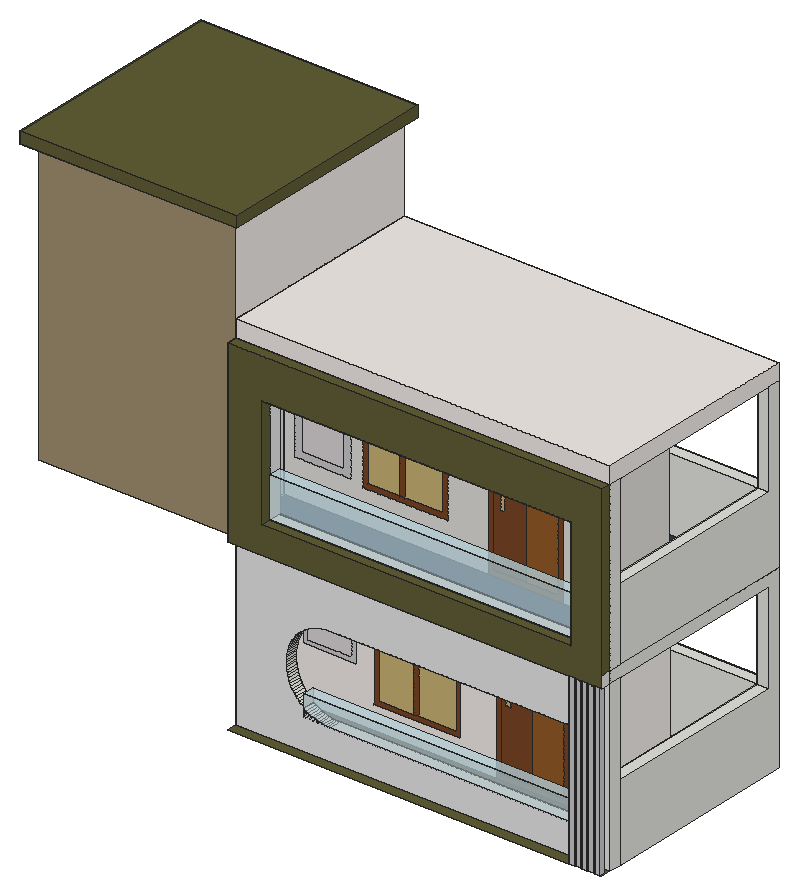
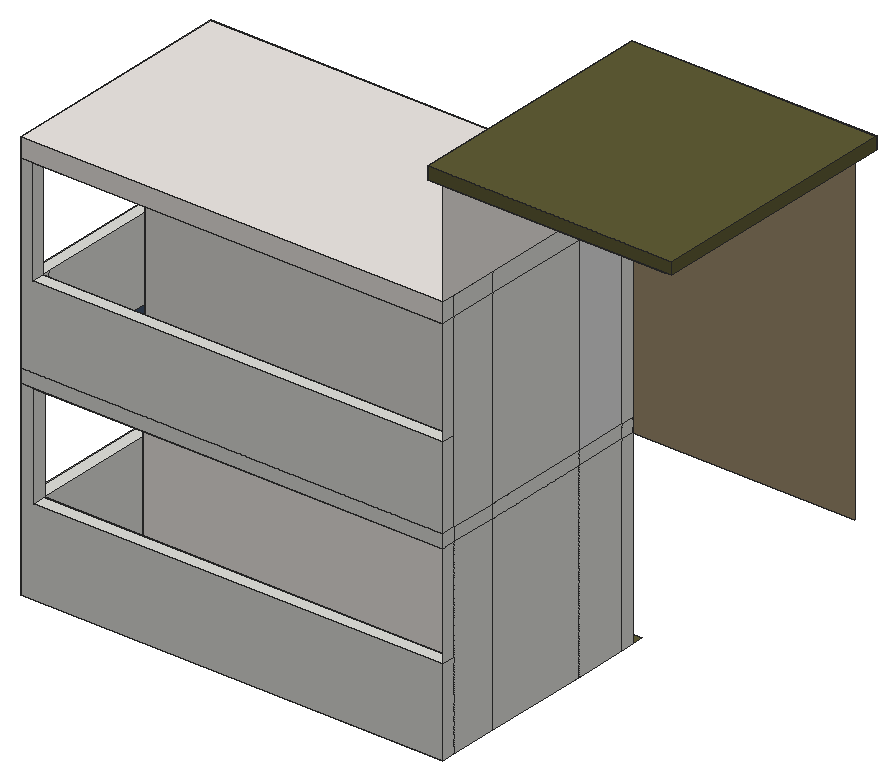
# SketchUp Ruby script. Lengths in inches.
U = 1.inch
M = Sketchup.active_model
def pt(a) = Geom::Point3d.new(a.map { |v| v * U })
def face(e, loops, mat)
  f = e.add_face(loops[0].map { |a| pt(a) })
  loops[1..].each { |l| e.add_face(l.map { |a| pt(a) }).erase! }
  f.material = f.back_material = mat if mat
  f
end
# faces: each face lists its corners as indices into pts; further lists are holes
def faces(e, pts, list, mat = nil) = list.each { |f| face(e, (f[0].is_a?(Array) ? f : [f]).map { |l| l.map { |i| pts[i] } }, mat) }
# xy, xz, yz: faces in a plane at the given z, y or x. An outline is a flat list of corners, or four numbers for a rectangle; further outlines are holes
def ring(l) = l.size == 4 ? [[l[0], l[1]], [l[2], l[1]], [l[2], l[3]], [l[0], l[3]]] : l.each_slice(2).to_a
def flat(e, list, mat, &to3) = list.each { |f| face(e, (f[0].is_a?(Array) ? f : [f]).map { |l| ring(l).map { |u, v| to3.(u, v) } }, mat) }
def xy(e, z, list, mat = nil) = flat(e, list, mat) { |x, y| [x, y, z] }
def xz(e, y, list, mat = nil) = flat(e, list, mat) { |x, z| [x, y, z] }
def yz(e, x, list, mat = nil) = flat(e, list, mat) { |y, z| [x, y, z] }
def lines(e, pts, list) = list.each { |a, b| e.add_line(pt(pts[a]), pt(pts[b])) }
# prism: a flat outline (further loops are holes) pulled along v
def prism(e, loops, v, mat = nil)
  f = face(e, loops, mat); d = Geom::Vector3d.new(v.map { |x| x * U })
  f.pushpull(f.normal.samedirection?(d) ? d.length : -d.length)
end
def box(e, o, s, mat = nil) = prism(e, [[o, [o[0] + s[0], o[1], o[2]], [o[0] + s[0], o[1] + s[1], o[2]], [o[0], o[1] + s[1], o[2]]]], [0, 0, s[2]], mat)
def at(x, y, z, deg = 0) = Geom::Transformation.translation(pt([x, y, z])) * Geom::Transformation.rotation(ORIGIN, Z_AXIS, deg.degrees)
def axes(o, x, y, z) = Geom::Transformation.new([*x, 0, *y, 0, *z, 0, *pt(o).to_a, 1])
def part(name) = M.definitions.add(name)
# library, detail: a bought-in or finely detailed component or shape, given as its bounding box
def library(name, o, s) = part(name).tap { |d| box(d.entities, o, s) }
def detail(e, o, s) = box(e.add_group.entities, o, s)
def put(e, d, t, mat = nil) = e.add_instance(d, t).tap { |i| i.material = mat if mat }
def group(e, t, mat = nil) = e.add_group.tap { |g| g.transformation = t; g.material = mat if mat }.entities
root = M.entities
M.materials.add("[0057_DarkKhaki]").color = [96, 93, 54]
M.materials.add("[Blinds Cellular White]").color = [217, 211, 213]
M.materials.add("[Leather Blue]").color = [45, 57, 74]
M.materials.add("[Leather Red Brown]").color = [76, 40, 8]
M.materials.add("[Polished Concrete New]").color = [200, 200, 203]
M.materials.add("[Polished Concrete Old]").color = [229, 229, 229]
M.materials.add("[Terrazzo Tile Accent]").color = [224, 221, 217]
M.materials.add("[Tile Border Travertine]").color = [160, 142, 112]
M.materials.add("[Translucent Glass Safety]").color = [204, 235, 244]
M.materials["[Translucent Glass Safety]"].alpha = 0.5
M.materials.add("[White Square Tile]").color = [240, 234, 230]
M.materials.add("[Window Covering 02]").color = [199, 178, 115]
M.materials.add("[Wood Floor Light]").color = [204, 176, 127]
M.materials.add("[Wood Floor Parquet]").color = [145, 89, 39]
M.materials.add("[Wood Veneer 01]").color = [120, 70, 37]
xy(root,986.8125,[[1036.87,294.37,1047.2,304.24],[1049.06,294.37,1059.38,304.24],[1060.68,294.37,1071.01,304.24],[1073.18,294.37,1083.51,304.24],[1085.87,294.37,1096.2,304.24],
  [386.67,314.12,1099.23,336.81],[1076.54,336.81,1076.54,692.27,386.67,692.27,386.67,714.96,1099.23,714.96,1099.23,336.81],[386.67,429.17,977.4,609.95]])
xy(root,986.8125,[[386.67,294.37,1036.87,294.37,1036.87,304.24,1047.2,304.24,1047.2,294.37,1049.06,294.37,1049.06,304.24,1059.38,304.24,1059.38,294.37,1060.68,294.37,1060.68,304.24,1071.01,304.24,1071.01,294.37,1073.18,294.37,1073.18,304.24,1083.51,304.24,1083.51,294.37,1085.87,294.37,1085.87,304.24,1096.2,304.24,1096.2,294.37,1099.23,294.37,1099.23,314.12,386.67,314.12]],"[0057_DarkKhaki]")
xy(root,986.8125,[[386.67,336.81,1076.54,336.81,1076.54,692.27,386.67,692.27,386.67,609.95,977.4,609.95,977.4,429.17,386.67,429.17]],"[Leather Red Brown]")
xy(root,1044.74,[[515.75,314.12,565.62,336.81],[565.62,314.12,1076.54,336.81]])
xy(root,1084.42,[[515.75,314.12,1076.54,336.81]],"[Translucent Glass Safety]")
xy(root,1132.25,[[1076.54,336.81,1099.23,692.27],[386.67,692.27,1076.54,714.96]])
xy(root,1210.05,[[565.62,314.12,1076.54,336.81]])
xy(root,1306.5625,[[1036.87,294.37,1047.2,295.05],[1049.06,294.37,1059.38,295.05],[1060.68,294.37,1071.01,295.05],[1073.18,294.37,1083.51,295.05],[1085.87,294.37,1096.2,295.05],
  [386.67,295.05,977.4,314.12],[977.4,295.05,977.4,314.12,1076.54,314.12,1076.54,304.24,1073.18,304.24,1073.18,295.05,1071.01,295.05,1071.01,304.24,1060.68,304.24,1060.68,295.05,1059.38,295.05,1059.38,304.24,1049.06,304.24,1049.06,295.05,1047.2,295.05,1047.2,304.24,1036.87,304.24,1036.87,295.05],[1036.87,295.05,1047.2,304.24],[1049.06,295.05,1059.38,304.24],[1060.68,295.05,1071.01,304.24],
  [1073.18,295.05,1076.54,304.24],[1076.54,295.05,1083.51,304.24],[1083.51,295.05,1083.51,304.24,1076.54,304.24,1076.54,314.12,1099.23,314.12,1099.23,295.05,1096.2,295.05,1096.2,304.24,1085.87,304.24,1085.87,295.05],[1085.87,295.05,1096.2,304.24],[386.67,314.12,977.4,336.81],
  [977.4,314.12,1076.54,336.81],[1076.54,314.12,1099.23,336.81],[386.67,336.81,1099.23,429.17],[386.67,429.17,977.4,609.95],[977.4,429.17,977.4,714.96,1076.54,714.96,1076.54,692.27,1099.23,692.27,1099.23,429.17],
  [386.67,609.95,977.4,714.96]])
xy(root,1329.25,[[1078.73,336.81,1078.73,692.27,386.67,692.27,386.67,714.96,1099.23,714.96,1099.23,336.81],[386.67,429.17,973.89,609.95]])
xy(root,1329.25,[[386.67,336.81,1078.73,336.81,1078.73,692.27,386.67,692.27,386.67,609.95,973.89,609.95,973.89,429.17,386.67,429.17]],"[Leather Blue]")
xy(root,1358.875,[[451.45,314.12,1039.41,336.81]])
xy(root,1358.875,[[451.45,295.05,1039.41,314.12]],"[0057_DarkKhaki]")
xy(root,1436.0625,[[451.45,314.12,1039.41,336.81]],"[Translucent Glass Safety]")
xy(root,1467.875,[[1078.73,336.81,1099.23,692.27],[386.67,692.27,1078.73,714.96]])
xy(root,1571.07,[[451.45,314.12,1039.41,336.81]])
xy(root,1571.07,[[451.45,295.05,1039.41,314.12]],"[0057_DarkKhaki]")
xy(root,1646.9375,[[386.67,336.81,1099.23,429.17],[386.67,429.17,973.89,609.95],[973.89,429.17,973.89,714.96,1078.73,714.96,1078.73,692.27,1099.23,692.27,1099.23,429.17],[386.67,609.95,973.89,714.96],[1078.73,692.27,1099.23,714.96]])
xy(root,1646.9375,[[386.67,295.05,1099.23,314.12]],"[0057_DarkKhaki]")
xy(root,1679.125,[[386.67,314.12,1099.23,714.96]],"[White Square Tile]")
xy(root,1855.8125,[[11.875,314.12,386.67,714.96]])
xy(root,1855.8125,[[0,284.3,0,314.12,386.67,314.12,386.67,714.96,412.48,714.96,412.48,284.3],[0,314.12,11.875,714.96]],"[0057_DarkKhaki]")
xy(root,1876.625,[[0,284.3,412.48,714.96]],"[0057_DarkKhaki]")
xz(root,284.3,[[0,1855.8125,412.48,1876.625]],"[0057_DarkKhaki]")
xz(root,294.37,[[1036.87,986.8125,1047.2,1306.5625],[1049.06,986.8125,1059.38,1306.5625],[1060.68,986.8125,1071.01,1306.5625],[1073.18,986.8125,1083.51,1306.5625],[1085.87,986.8125,1096.2,1306.5625]],"[Polished Concrete New]")
xz(root,295.05,[[[386.67,1306.5625,1099.23,1646.9375],[451.45,1358.875,1039.41,1571.07]]],"[0057_DarkKhaki]")
xz(root,304.24,[[1036.87,986.8125,1047.2,1306.5625],[1049.06,986.8125,1059.38,1306.5625],[1060.68,986.8125,1071.01,1306.5625],[1073.18,986.8125,1083.51,1306.5625],[1085.87,986.8125,1096.2,1306.5625]])
xz(root,314.12,[[515.75,1044.74,565.62,1044.74,561.3,1044.85,556.98,1045.1875,552.69,1045.75,548.4375,1046.54,544.23,1047.55,540.08,1048.78,538.62,1049.3,515.75,1049.3],[515.75,1049.3,538.62,1049.3,536,1050.23,532,1051.88,528.1,1053.74,524.29,1055.81,520.6,1058.07,517.04,1060.52,515.75,1061.51],[[386.67,1306.5625,1099.23,1646.9375],[451.45,1358.875,1039.41,1571.07]]])
xz(root,314.12,[[[386.67,986.8125,1099.23,1306.5625],[565.62,1044.74,561.3,1044.85,556.98,1045.1875,552.69,1045.75,548.4375,1046.54,544.23,1047.55,540.08,1048.78,538.62,1049.3,536,1050.23,532,1051.88,528.1,1053.74,524.29,1055.81,520.6,1058.07,517.04,1060.52,513.6,1063.16,510.3125,1065.97,507.17,1068.94,504.2,1072.08,501.38,1075.375,498.75,1078.81,496.3,1082.375,494.04,1086.0625,491.97,1089.87,490.11,1093.77,488.45,1097.77,487.01,1101.85,485.78,1106,484.77,1110.21,483.98,1114.46,483.42,1118.75,483.08,1123.07,482.96,1127.39,483.08,1131.72,483.42,1136.03,483.98,1140.32,484.77,1144.58,485.78,1148.78,487.01,1152.93,488.45,1157.01,490.11,1161.01,491.97,1164.92,494.04,1168.72,496.3,1172.41,498.75,1175.98,501.38,1179.41,504.2,1182.7,507.17,1185.84,510.3125,1188.82,513.6,1191.63,517.04,1194.26,520.6,1196.71,524.29,1198.97,528.1,1201.04,532,1202.9,536,1204.56,540.08,1206,544.23,1207.23,548.4375,1208.24,552.69,1209.03,556.98,1209.59,561.3,1209.93,565.62,1210.05,1076.54,1210.05,1076.54,1044.74]]],"[Polished Concrete Old]")
xz(root,314.12,[[11.875,1306.5625,386.67,1855.8125]],"[Tile Border Travertine]")
xz(root,314.12,[[565.62,1044.74,1076.54,1044.74,1076.54,1084.42,515.75,1084.42,515.75,1061.51,517.04,1060.52,520.6,1058.07,524.29,1055.81,528.1,1053.74,532,1051.88,536,1050.23,538.62,1049.3,540.08,1048.78,544.23,1047.55,548.4375,1046.54,552.69,1045.75,556.98,1045.1875,561.3,1044.85],[451.45,1358.875,1039.41,1436.0625]],"[Translucent Glass Safety]")
xz(root,314.12,[[386.67,1646.9375,1099.23,1679.125]],"[White Square Tile]")
xz(root,336.81,[[386.67,986.8125,386.67,1306.5625,1076.54,1306.5625,1076.54,1210.05,565.62,1210.05,561.3,1209.93,556.98,1209.59,552.69,1209.03,548.4375,1208.24,544.23,1207.23,540.08,1206,536,1204.56,532,1202.9,528.1,1201.04,524.29,1198.97,520.6,1196.71,517.04,1194.26,513.6,1191.63,510.3125,1188.82,507.17,1185.84,504.2,1182.7,501.38,1179.41,498.75,1175.98,496.3,1172.41,494.04,1168.72,491.97,1164.92,490.11,1161.01,488.45,1157.01,487.01,1152.93,485.78,1148.78,484.77,1144.58,483.98,1140.32,483.42,1136.03,483.08,1131.72,482.96,1127.39,483.08,1123.07,483.42,1118.75,483.98,1114.46,484.77,1110.21,485.78,1106,487.01,1101.85,488.45,1097.77,490.11,1093.77,491.97,1089.87,494.04,1086.0625,496.3,1082.375,498.75,1078.81,501.38,1075.375,504.2,1072.08,507.17,1068.94,510.3125,1065.97,513.6,1063.16,515.75,1061.51,515.75,1044.74,1076.54,1044.74,1076.54,986.8125],[1076.54,986.8125,1099.23,1132.25],[515.75,1044.74,515.75,1049.3,538.62,1049.3,540.08,1048.78,544.23,1047.55,548.4375,1046.54,552.69,1045.75,556.98,1045.1875,561.3,1044.85,565.62,1044.74],[515.75,1049.3,515.75,1061.51,517.04,1060.52,520.6,1058.07,524.29,1055.81,528.1,1053.74,532,1051.88,536,1050.23,538.62,1049.3],[1076.54,1132.25,1099.23,1306.5625],
  [386.67,1329.25,386.67,1646.9375,1078.73,1646.9375,1078.73,1329.25,1039.41,1329.25,1039.41,1571.07,451.45,1571.07,451.45,1329.25],[451.45,1329.25,1039.41,1358.875],[1078.73,1329.25,1099.23,1467.875],[1078.73,1467.875,1099.23,1646.9375]])
xz(root,336.81,[[565.62,1044.74,561.3,1044.85,556.98,1045.1875,552.69,1045.75,548.4375,1046.54,544.23,1047.55,540.08,1048.78,538.62,1049.3,536,1050.23,532,1051.88,528.1,1053.74,524.29,1055.81,520.6,1058.07,517.04,1060.52,515.75,1061.51,515.75,1084.42,1076.54,1084.42,1076.54,1044.74],[451.45,1358.875,1039.41,1436.0625]],"[Translucent Glass Safety]")
xz(root,429.17,[[431.13,1097.14,515.01,1252.02],[419.91,1413.17,499.9,1575.28]],"[Blinds Cellular White]")
xz(root,429.17,[[[421.45,1087.45,524.7,1261.7],[431.13,1097.14,515.01,1252.02]],[[406.97,1400.22,512.84,1588.22],[419.91,1413.17,499.9,1575.28]]],"[Polished Concrete New]")
xz(root,429.17,[[[386.67,1329.25,774.49,1329.25,774.49,1604.375,918.87,1604.375,918.87,1329.25,973.89,1329.25,973.89,1646.9375,386.67,1646.9375],[536.93,1393.05,698.24,1572.36],[406.97,1400.22,512.84,1588.22]]],"[Terrazzo Tile Accent]")
xz(root,429.17,[[[386.67,986.8125,789.43,986.8125,789.43,1274.3125,930.49,1274.3125,930.49,986.8125,977.4,986.8125,977.4,1306.5625,386.67,1306.5625],[557.89,1030.65,723.33,1218.09],[421.45,1087.45,524.7,1261.7]]],"[White Square Tile]")
xz(root,429.17,[[568.01,1040.77,634.54,1207.97],[643.33,1040.77,713.21,1207.97],[546.9,1403.01,607.25,1562.39],[616.99,1403.01,688.28,1562.39]],"[Window Covering 02]")
xz(root,429.17,[[809.05,1116.57,817.99,1168.76],[798.86,1447.23,807.55,1494.6]],"[Wood Floor Light]")
xz(root,429.17,[[859.96,997.33,919.97,1263.8],[846.68,1341.08,907.04,1592.54]],"[Wood Floor Parquet]")
xz(root,429.17,[[[789.43,986.8125,930.49,1274.3125],[799.94,997.33,919.97,1263.8]],[[799.94,997.33,859.96,1263.8],[809.05,1116.57,817.99,1168.76]],[[557.89,1030.65,723.33,1218.09],[568.01,1040.77,713.21,1207.97]],[634.54,1040.77,643.33,1207.97],[[774.49,1329.25,918.87,1604.375],[786.33,1341.08,907.04,1592.54]],
  [[786.33,1341.08,846.68,1592.54],[798.86,1447.23,807.55,1494.6]],[[536.93,1393.05,698.24,1572.36],[546.9,1403.01,688.28,1562.39]],[607.25,1403.01,616.99,1562.39]],"[Wood Veneer 01]")
xz(root,609.95,[[386.67,1329.25,973.89,1646.9375]],"[Terrazzo Tile Accent]")
xz(root,609.95,[[386.67,986.8125,977.4,1306.5625]],"[White Square Tile]")
xz(root,692.27,[[386.67,986.8125,1076.54,1132.25],[1076.54,1132.25,1099.23,1306.5625],[386.67,1329.25,1078.73,1467.875],[1078.73,1467.875,1099.23,1646.9375]])
xz(root,714.96,[[386.67,986.8125,386.67,1132.25,1076.54,1132.25,1076.54,1306.5625,1099.23,1306.5625,1099.23,986.8125],[386.67,1306.5625,1099.23,1329.25],[386.67,1329.25,386.67,1467.875,1078.73,1467.875,1078.73,1646.9375,1099.23,1646.9375,1099.23,1329.25]])
xz(root,714.96,[[0,1855.8125,412.48,1876.625]],"[0057_DarkKhaki]")
xz(root,714.96,[[386.67,1646.9375,1099.23,1679.125]],"[White Square Tile]")
yz(root,0,[[284.3,1855.8125,714.96,1876.625]],"[0057_DarkKhaki]")
yz(root,386.67,[[314.12,986.8125,336.81,1306.5625],[336.81,986.8125,429.17,1306.5625],[429.17,986.8125,609.95,1306.5625],[609.95,986.8125,692.27,1306.5625],[692.27,986.8125,714.96,1132.25],
  [692.27,1132.25,714.96,1306.5625],[314.12,1306.5625,336.81,1329.25],[336.81,1306.5625,429.17,1329.25],[429.17,1306.5625,609.95,1329.25],[609.95,1306.5625,692.27,1329.25],
  [692.27,1306.5625,714.96,1329.25],[314.12,1329.25,336.81,1679.125],[429.17,1329.25,609.95,1646.9375],[609.95,1329.25,692.27,1646.9375],[692.27,1329.25,714.96,1467.875],
  [692.27,1467.875,714.96,1646.9375],[336.81,1646.9375,429.17,1679.125],[429.17,1646.9375,609.95,1679.125],[609.95,1646.9375,692.27,1679.125],[692.27,1646.9375,714.96,1679.125]])
yz(root,386.67,[[295.05,1306.5625,314.12,1646.9375]],"[0057_DarkKhaki]")
yz(root,386.67,[[336.81,1329.25,429.17,1646.9375]],"[Polished Concrete Old]")
yz(root,386.67,[[314.12,1679.125,714.96,1855.8125]],"[White Square Tile]")
yz(root,412.48,[[284.3,1855.8125,714.96,1876.625]],"[0057_DarkKhaki]")
yz(root,451.45,[[314.12,1358.875,336.81,1436.0625]])
yz(root,451.45,[[295.05,1358.875,314.12,1571.07]],"[0057_DarkKhaki]")
yz(root,451.45,[[314.12,1436.0625,336.81,1571.07]],"[Polished Concrete Old]")
yz(root,515.75,[[314.12,1044.74,336.81,1084.42]])
yz(root,973.89,[[429.17,1329.25,609.95,1646.9375]],"[Terrazzo Tile Accent]")
yz(root,977.4,[[429.17,986.8125,609.95,1306.5625]],"[White Square Tile]")
yz(root,1036.87,[[294.37,986.8125,304.24,1306.5625]],"[Polished Concrete New]")
yz(root,1039.41,[[314.12,1358.875,336.81,1436.0625]])
yz(root,1039.41,[[295.05,1358.875,314.12,1571.07]],"[0057_DarkKhaki]")
yz(root,1039.41,[[314.12,1436.0625,336.81,1571.07]],"[Polished Concrete Old]")
yz(root,1047.2,[[294.37,986.8125,304.24,1306.5625]],"[Polished Concrete New]")
yz(root,1049.06,[[294.37,986.8125,304.24,1306.5625]])
yz(root,1059.38,[[294.37,986.8125,304.24,1306.5625]],"[Polished Concrete New]")
yz(root,1060.68,[[294.37,986.8125,304.24,1306.5625]])
yz(root,1071.01,[[294.37,986.8125,304.24,1306.5625]],"[Polished Concrete New]")
yz(root,1073.18,[[294.37,986.8125,304.24,1306.5625]])
yz(root,1076.54,[[336.81,986.8125,692.27,1132.25],[314.12,1044.74,336.81,1084.42],[314.12,1084.42,336.81,1210.05],[692.27,1132.25,714.96,1306.5625]])
yz(root,1078.73,[[336.81,1329.25,679.87,1467.875],[679.87,1329.25,692.27,1467.875],[692.27,1467.875,714.96,1646.9375]])
yz(root,1083.51,[[294.37,986.8125,304.24,1306.5625]],"[Polished Concrete New]")
yz(root,1085.87,[[294.37,986.8125,304.24,1306.5625]])
yz(root,1096.2,[[294.37,986.8125,304.24,1306.5625]],"[Polished Concrete New]")
yz(root,1099.23,[[314.12,986.8125,336.81,1306.5625],[336.81,986.8125,714.96,986.8125,714.96,1329.25,314.12,1329.25,314.12,1306.5625,692.27,1306.5625,692.27,1132.25,336.81,1132.25],[295.05,1306.5625,314.12,1329.25],[314.12,1329.25,336.81,1646.9375],[336.81,1329.25,714.96,1329.25,714.96,1646.9375,692.27,1646.9375,692.27,1467.875,336.81,1467.875]])
yz(root,1099.23,[[295.05,1329.25,314.12,1646.9375]],"[0057_DarkKhaki]")
yz(root,1099.23,[[314.12,1646.9375,714.96,1679.125]],"[White Square Tile]")
p = [[561.3,314.12,1044.85],[565.62,314.12,1044.74],[565.62,336.81,1044.74],[561.3,336.81,1044.85],[556.98,314.12,1045.1875],[556.98,336.81,1045.1875],
  [552.69,314.12,1045.75],[552.69,336.81,1045.75],[548.4375,314.12,1046.54],[548.4375,336.81,1046.54],[544.23,314.12,1047.55],[544.23,336.81,1047.55],
  [540.08,314.12,1048.78],[540.08,336.81,1048.78],[536,314.12,1050.23],[538.62,314.12,1049.3],[538.62,336.81,1049.3],[536,336.81,1050.23],
  [532,314.12,1051.88],[532,336.81,1051.88],[528.1,314.12,1053.74],[528.1,336.81,1053.74],[524.29,314.12,1055.81],[524.29,336.81,1055.81],
  [520.6,314.12,1058.07],[520.6,336.81,1058.07],[517.04,314.12,1060.52],[517.04,336.81,1060.52],[513.6,314.12,1063.16],[515.75,314.12,1061.51],
  [515.75,336.81,1061.51],[513.6,336.81,1063.16],[510.3125,314.12,1065.97],[510.3125,336.81,1065.97],[507.17,314.12,1068.94],[507.17,336.81,1068.94],
  [504.2,314.12,1072.08],[504.2,336.81,1072.08],[501.38,314.12,1075.375],[501.38,336.81,1075.375],[498.75,314.12,1078.81],[498.75,336.81,1078.81],
  [496.3,314.12,1082.375],[496.3,336.81,1082.375],[494.04,314.12,1086.0625],[494.04,336.81,1086.0625],[491.97,314.12,1089.87],[491.97,336.81,1089.87],
  [490.11,314.12,1093.77],[490.11,336.81,1093.77],[488.45,314.12,1097.77],[488.45,336.81,1097.77],[487.01,314.12,1101.85],[487.01,336.81,1101.85],
  [485.78,314.12,1106],[485.78,336.81,1106],[484.77,314.12,1110.21],[484.77,336.81,1110.21],[483.98,314.12,1114.46],[483.98,336.81,1114.46],
  [483.42,314.12,1118.75],[483.42,336.81,1118.75],[483.08,314.12,1123.07],[483.08,336.81,1123.07],[482.96,314.12,1127.39],[482.96,336.81,1127.39],
  [483.08,314.12,1131.72],[483.08,336.81,1131.72],[483.42,314.12,1136.03],[483.42,336.81,1136.03],[483.98,314.12,1140.32],[483.98,336.81,1140.32],
  [484.77,314.12,1144.58],[484.77,336.81,1144.58],[485.78,314.12,1148.78],[485.78,336.81,1148.78],[487.01,314.12,1152.93],[487.01,336.81,1152.93],
  [488.45,314.12,1157.01],[488.45,336.81,1157.01],[490.11,314.12,1161.01],[490.11,336.81,1161.01],[491.97,314.12,1164.92],[491.97,336.81,1164.92],
  [494.04,314.12,1168.72],[494.04,336.81,1168.72],[496.3,314.12,1172.41],[496.3,336.81,1172.41],[498.75,314.12,1175.98],[498.75,336.81,1175.98],
  [501.38,314.12,1179.41],[501.38,336.81,1179.41],[504.2,314.12,1182.7],[504.2,336.81,1182.7],[507.17,314.12,1185.84],[507.17,336.81,1185.84],
  [510.3125,314.12,1188.82],[510.3125,336.81,1188.82],[513.6,314.12,1191.63],[513.6,336.81,1191.63],[517.04,314.12,1194.26],[517.04,336.81,1194.26],
  [520.6,314.12,1196.71],[520.6,336.81,1196.71],[524.29,314.12,1198.97],[524.29,336.81,1198.97],[528.1,314.12,1201.04],[528.1,336.81,1201.04],
  [532,314.12,1202.9],[532,336.81,1202.9],[536,314.12,1204.56],[536,336.81,1204.56],[540.08,314.12,1206],[540.08,336.81,1206],
  [544.23,314.12,1207.23],[544.23,336.81,1207.23],[548.4375,314.12,1208.24],[548.4375,336.81,1208.24],[552.69,314.12,1209.03],[552.69,336.81,1209.03],
  [556.98,314.12,1209.59],[556.98,336.81,1209.59],[561.3,314.12,1209.93],[561.3,336.81,1209.93],[565.62,314.12,1210.05],[565.62,336.81,1210.05],
  [1039.41,314.12,1329.25],[1039.41,336.81,1329.25],[451.45,314.12,1329.25],[451.45,336.81,1329.25]]
faces(root,p,[[0,1,2,3],[4,0,3,5],[6,4,5,7],[8,6,7,9],[10,8,9,11],[12,10,11,13],[14,15,12,13,16,17],[18,14,17,19],
  [20,18,19,21],[22,20,21,23],[24,22,23,25],[26,24,25,27],[28,29,26,27,30,31],[32,28,31,33],[34,32,33,35],[36,34,35,37],
  [38,36,37,39],[40,38,39,41],[42,40,41,43],[44,42,43,45],[46,44,45,47],[48,46,47,49],[50,48,49,51],[52,50,51,53],
  [54,52,53,55],[56,54,55,57],[58,56,57,59],[60,58,59,61],[62,60,61,63],[64,62,63,65],[66,64,65,67],[68,66,67,69],
  [70,68,69,71],[72,70,71,73],[74,72,73,75],[76,74,75,77],[78,76,77,79],[80,78,79,81],[82,80,81,83],[84,82,83,85],
  [86,84,85,87],[88,86,87,89],[90,88,89,91],[92,90,91,93],[94,92,93,95],[96,94,95,97],[98,96,97,99],[100,98,99,101],
  [102,100,101,103],[104,102,103,105],[106,104,105,107],[108,106,107,109],[110,108,109,111],[112,110,111,113],[114,112,113,115],[116,114,115,117],
  [118,116,117,119],[120,118,119,121],[122,120,121,123],[124,122,123,125]])
lines(root,p,[[126,127],[128,129]])
